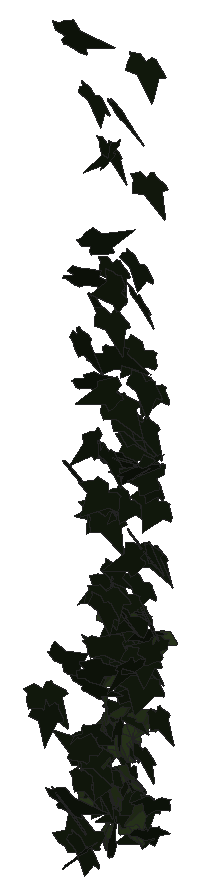
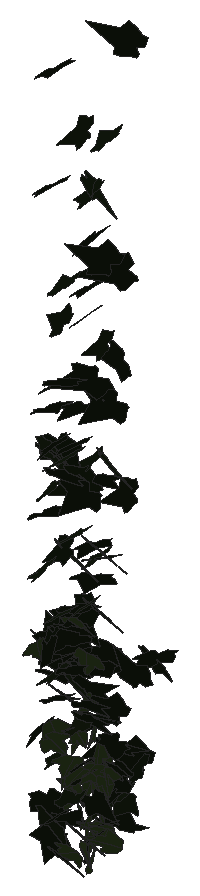
# SketchUp Ruby script. Lengths in inches.
U = 1.inch
M = Sketchup.active_model
def pt(a) = Geom::Point3d.new(a.map { |v| v * U })
def face(e, loops, mat)
  f = e.add_face(loops[0].map { |a| pt(a) })
  loops[1..].each { |l| e.add_face(l.map { |a| pt(a) }).erase! }
  f.material = f.back_material = mat if mat
  f
end
# faces: each face lists its corners as indices into pts; further lists are holes
def faces(e, pts, list, mat = nil) = list.each { |f| face(e, (f[0].is_a?(Array) ? f : [f]).map { |l| l.map { |i| pts[i] } }, mat) }
# xy, xz, yz: faces in a plane at the given z, y or x. An outline is a flat list of corners, or four numbers for a rectangle; further outlines are holes
def ring(l) = l.size == 4 ? [[l[0], l[1]], [l[2], l[1]], [l[2], l[3]], [l[0], l[3]]] : l.each_slice(2).to_a
def flat(e, list, mat, &to3) = list.each { |f| face(e, (f[0].is_a?(Array) ? f : [f]).map { |l| ring(l).map { |u, v| to3.(u, v) } }, mat) }
def xy(e, z, list, mat = nil) = flat(e, list, mat) { |x, y| [x, y, z] }
def xz(e, y, list, mat = nil) = flat(e, list, mat) { |x, z| [x, y, z] }
def yz(e, x, list, mat = nil) = flat(e, list, mat) { |y, z| [x, y, z] }
def lines(e, pts, list) = list.each { |a, b| e.add_line(pt(pts[a]), pt(pts[b])) }
# prism: a flat outline (further loops are holes) pulled along v
def prism(e, loops, v, mat = nil)
  f = face(e, loops, mat); d = Geom::Vector3d.new(v.map { |x| x * U })
  f.pushpull(f.normal.samedirection?(d) ? d.length : -d.length)
end
def box(e, o, s, mat = nil) = prism(e, [[o, [o[0] + s[0], o[1], o[2]], [o[0] + s[0], o[1] + s[1], o[2]], [o[0], o[1] + s[1], o[2]]]], [0, 0, s[2]], mat)
def at(x, y, z, deg = 0) = Geom::Transformation.translation(pt([x, y, z])) * Geom::Transformation.rotation(ORIGIN, Z_AXIS, deg.degrees)
def axes(o, x, y, z) = Geom::Transformation.new([*x, 0, *y, 0, *z, 0, *pt(o).to_a, 1])
def part(name) = M.definitions.add(name)
# library, detail: a bought-in or finely detailed component or shape, given as its bounding box
def library(name, o, s) = part(name).tap { |d| box(d.entities, o, s) }
def detail(e, o, s) = box(e.add_group.entities, o, s)
def put(e, d, t, mat = nil) = e.add_instance(d, t).tap { |i| i.material = mat if mat }
def group(e, t, mat = nil) = e.add_group.tap { |g| g.transformation = t; g.material = mat if mat }.entities
root = M.entities
M.materials.add("1026 AP 7946 SUNNY SIDE UP").color = [254, 231, 186]
M.materials.add("efeu1").color = [18, 25, 13]
M.materials.add("efeu2").color = [43, 57, 29]
c1 = part("ivyleaf_9")
p = [[1.54,2.16,1.25],[1.36,2.04,1.19],[-0.21,0.99,0.68],[-0.71,1.11,0.82],[-0.85,0.86,0.67],[-0.8,0.17,0.21],
  [-0.9,-0.01,0.1],[-0.67,-0.16,-0.02],[-0.08,-0.08,-0.05],[-0.03,-0.6,-0.4],[0.65,-0.88,-0.66],[0.83,-0.6,-0.49],
  [1.29,-0.42,-0.43],[1.8125,-0.07,-0.26],[1.21,0.44,0.15]]
faces(c1.entities,p,[[0,1,2,3,4,5,6,7,8,9,10,11,12,13,14]],"efeu1")
c2 = part("ivyleaf_10")
p = [[0,0.5,-0.03],[-0.0625,2.02,-0.43],[-0.19,2.01,-0.46],[-0.54,1.05,-0.29],[-0.52,0.625,-0.18],[-0.83,0.76,-0.28],
  [-1.16,0.64,-0.33],[-1.15,0.33,-0.24],[-0.77,-0.39,0.02],[-0.3,-0.51,0.16],[0.04,-0.48,0.23],[-0.02,2.01,-0.4375],
  [-0.06,2.01,-0.43],[0.04,-0.49,0.23],[0.67,-0.49,0.14],[1.38,0.36,-0.2],[1.375,0.51,-0.24],[0.81,0.65,-0.19],
  [0.62,0.59,-0.15],[0.6,1.09,-0.28],[0.5,1.23,-0.31]]
faces(c2.entities,p,[[0,1,2,3,4,5,6,7,8,9,10],[11,12,0,13,14,15,16,17,18,19,20]],"efeu2")
put(root,c1,axes([142.15,210.58,305.85],[0.56182,-0.24901,0.07476],[0.06155,-0.07277,-0.44748],[0.40379,0.35755,-0.03581]),"1026 AP 7946 SUNNY SIDE UP")
put(root,c1,axes([142.23,210.13,298.04],[-0.16216,0.04848,0.41407],[0.43975,-0.29098,0.10846],[0.45969,0.29546,0.04232]),"1026 AP 7946 SUNNY SIDE UP")
put(root,c2,axes([142.22,211.47,291.9],[-0.09766,-0.0032,0.39572],[0.44557,0.26235,0.05098],[-0.40784,0.28739,-0.03905]),"1026 AP 7946 SUNNY SIDE UP")
put(root,c1,axes([142.65,211.97,303.67],[-0.39464,-0.2842,0.1348],[0.01517,-0.17659,-0.37252],[0.4928,-0.22216,0.11942]),"1026 AP 7946 SUNNY SIDE UP")
put(root,c1,axes([142.35,211.77,320.69],[0.01203,-0.38419,0.25002],[0.09974,-0.24162,-0.394],[0.7094,0.04049,0.05115]),"1026 AP 7946 SUNNY SIDE UP")
put(root,c2,axes([142.7,211.37,294.5625],[-0.1224,-0.38129,-0.03837],[0.00721,0.03487,-0.4007],[0.60204,-0.07794,-0.00301]),"1026 AP 7946 SUNNY SIDE UP")
put(root,c1,axes([142.92,211.75,293.68],[-0.17105,0.24532,-0.2627],[0.04053,-0.26199,-0.27106],[-0.5565,-0.09449,0.061]),"1026 AP 7946 SUNNY SIDE UP")
put(root,c1,axes([142.77,211.86,292.65],[-0.37015,-0.23425,0.17707],[-0.05585,-0.19795,-0.32668],[0.45467,-0.21501,0.10402]),"1026 AP 7946 SUNNY SIDE UP")
put(root,c1,axes([143,212.11,297.29],[-0.56008,-0.05361,0.10937],[-0.12492,-0.14335,-0.34901],[0.13974,-0.34301,0.12636]),"1026 AP 7946 SUNNY SIDE UP")
put(root,c1,axes([143.2,211.61,303.96],[-0.52628,0.24654,0.09131],[-0.15815,0.00943,-0.42496],[-0.37958,-0.34575,0.05046]),"1026 AP 7946 SUNNY SIDE UP")
put(root,c1,axes([142.41,211.6875,312.36],[0.43938,-0.32096,0.01476],[-0.01385,-0.02904,-0.43778],[0.50513,0.27839,-0.02484]),"1026 AP 7946 SUNNY SIDE UP")
put(root,c1,axes([142.96,212.32,297.8],[-0.52887,-0.16853,0.03592],[-0.02311,-0.05023,-0.38586],[0.26994,-0.3345,0.03735]),"1026 AP 7946 SUNNY SIDE UP")
put(root,c2,axes([143.05,211.21,294.29],[-0.49013,0.10462,0.18163],[-0.27752,0.02416,-0.33723],[-0.16241,-0.357,0.02813]),"1026 AP 7946 SUNNY SIDE UP")
put(root,c2,axes([142.87,211.92,294.82],[0.22328,0.24384,-0.27449],[-0.17662,-0.24385,-0.29149],[-0.54146,0.18009,-0.01811]),"1026 AP 7946 SUNNY SIDE UP")
put(root,c1,axes([143.05,212.14,297.15],[-0.57967,-0.07156,-0.00169],[0.01229,-0.03379,-0.38542],[0.11186,-0.3671,0.03356]),"1026 AP 7946 SUNNY SIDE UP")
put(root,c1,axes([142.94,211.03,294.74],[-0.5539,-0.10903,-0.12035],[0.18925,0.00271,-0.37848],[0.1642,-0.37092,0.03025]),"1026 AP 7946 SUNNY SIDE UP")
put(root,c1,axes([143.15,210.9,307.13],[-0.58674,0.18478,-0.14982],[0.17748,-0.10077,-0.42777],[-0.32553,-0.38799,0.03682]),"1026 AP 7946 SUNNY SIDE UP")
put(root,c2,axes([142.49,211.59,292.5],[0.05579,-0.14515,-0.35271],[0.58133,0.04364,0.02072],[0.05071,-0.3406,0.15058]),"1026 AP 7946 SUNNY SIDE UP")
put(root,c1,axes([143.24,211.65,318.73],[-0.47623,0.33135,-0.12901],[0.10289,-0.11211,-0.46233],[-0.54848,-0.30874,0.02529]),"1026 AP 7946 SUNNY SIDE UP")
put(root,c1,axes([142.47,210.72,311.3],[-0.00696,-0.0332,-0.47585],[0.72787,0.00217,-0.00472],[0.00393,-0.46173,0.03147]),"1026 AP 7946 SUNNY SIDE UP")
put(root,c2,axes([143.09,211.16,292.66],[0.23101,-0.30684,-0.17315],[-0.10165,0.15342,-0.3495],[0.53931,0.16035,0.00829]),"1026 AP 7946 SUNNY SIDE UP")
put(root,c2,axes([143.02,211.08,294.53],[0.09477,0.20416,-0.33964],[-0.15232,-0.31635,-0.22114],[-0.59201,0.11408,0.00253]),"1026 AP 7946 SUNNY SIDE UP")
put(root,c1,axes([142.97,211.62,292.02],[-0.17279,-0.25937,0.22693],[-0.09181,-0.21523,-0.29042],[0.52865,-0.12216,0.02373]),"1026 AP 7946 SUNNY SIDE UP")
put(root,c1,axes([142.71,210.875,309.56],[0.55799,0.25387,0.14941],[0.21938,0.05084,-0.44751],[-0.40273,0.37943,-0.03676]),"1026 AP 7946 SUNNY SIDE UP")
put(root,c1,axes([142.39,210.16,323.9],[0.25932,-0.02808,0.45404],[0.61742,-0.20636,-0.16606],[0.31836,0.42309,-0.04779]),"1026 AP 7946 SUNNY SIDE UP")
put(root,c1,axes([143.47,209.95,294.84],[-0.1309,0.16315,0.34222],[-0.53841,0.09301,-0.1353],[-0.21736,-0.32866,0.12904]),"1026 AP 7946 SUNNY SIDE UP")
put(root,c2,axes([143.02,211.31,295.42],[0.00064,-0.32487,-0.19179],[0.05825,0.18345,-0.33193],[0.58442,-0.01793,0.0333]),"1026 AP 7946 SUNNY SIDE UP")
put(root,c1,axes([142.81,210.5625,293.5],[0.18628,-0.37561,-0.22452],[-0.13524,0.19889,-0.40408],[0.6676,0.1451,-0.01921]),"1026 AP 7946 SUNNY SIDE UP")
put(root,c1,axes([142.68,212.14,318.62],[0.28861,-0.40925,0.05953],[0.01196,-0.06241,-0.46204],[0.65029,0.18278,-0.01792]),"1026 AP 7946 SUNNY SIDE UP")
put(root,c1,axes([143.48,211.49,297.87],[-0.00745,0.14018,0.37491],[-0.57798,0.11785,-0.05112],[-0.20134,-0.3435,0.13288]),"1026 AP 7946 SUNNY SIDE UP")
put(root,c1,axes([142.54,210.51,294.08],[0.35755,0.10931,-0.31997],[0.41372,0.16786,0.25977],[0.31279,-0.34697,0.02216]),"1026 AP 7946 SUNNY SIDE UP")
put(root,c1,axes([142.8,212.28,313.67],[0.11444,-0.43428,-0.01193],[-0.00085,0.00915,-0.45357],[0.68301,0.07278,0.00143]),"1026 AP 7946 SUNNY SIDE UP")
put(root,c1,axes([142.55,210.9375,296.875],[0.19017,-0.11545,0.38404],[0.52678,-0.17077,-0.16716],[0.31664,0.35344,0.04745]),"1026 AP 7946 SUNNY SIDE UP")
put(root,c2,axes([143.12,210.79,294.86],[0.20138,-0.37363,0.07668],[0.01933,-0.07667,-0.40712],[0.59939,0.128,-0.01264]),"1026 AP 7946 SUNNY SIDE UP")
put(root,c1,axes([143.41,211.23,301.14],[-0.6215,0.11195,-0.05232],[0.05893,-0.05534,-0.42124],[-0.18452,-0.39472,0.04168]),"1026 AP 7946 SUNNY SIDE UP")
put(root,c1,axes([142.88,208.1875,298.01],[0.02358,-0.36781,-0.3025],[0.06117,0.29167,-0.3753],[0.73546,-0.01246,0.04091]),"1026 AP 7946 SUNNY SIDE UP")
put(root,c2,axes([143.05,211.95,299.5],[0.61704,0.00807,0.06382],[0.09665,0.01891,-0.40384],[-0.01715,0.39682,0.02028]),"1026 AP 7946 SUNNY SIDE UP")
put(root,c2,axes([143.29,211.15,293.8],[0.07042,-0.38256,0.03993],[0.0033,-0.04096,-0.39703],[0.60496,0.04475,-0.00248]),"1026 AP 7946 SUNNY SIDE UP")
put(root,c1,axes([143.04,210.33,295.3],[0.09394,0.01372,-0.42097],[-0.04812,0.41204,0.01206],[0.64121,0.02891,0.06258]),"1026 AP 7946 SUNNY SIDE UP")
put(root,c2,axes([143.34,211.47,292.61],[-0.1965,0.34061,0.13927],[-0.15386,0.10455,-0.36923],[-0.55413,-0.14981,0.05313]),"1026 AP 7946 SUNNY SIDE UP")
put(root,c2,axes([143.42,211.39,290.625],[-0.24085,0.33001,-0.08377],[-0.04459,0.07854,0.3752],[0.53329,0.15561,-0.00646]),"1026 AP 7946 SUNNY SIDE UP")
put(root,c2,axes([143.34,211.79,297.35],[0.05907,0.14871,-0.37206],[-0.13408,-0.35182,-0.16006],[-0.60058,0.09317,-0.00086]),"1026 AP 7946 SUNNY SIDE UP")
put(root,c2,axes([143.36,211.16,296.12],[0.15168,-0.19433,-0.35009],[0.01038,0.34967,-0.20269],[0.61395,0.0421,0.08992]),"1026 AP 7946 SUNNY SIDE UP")
put(root,c1,axes([142.94,210.93,315.14],[0.05738,-0.02267,0.47504],[0.68454,0.15606,-0.02667],[-0.24227,0.43558,0.03716]),"1026 AP 7946 SUNNY SIDE UP")
put(root,c1,axes([143.63,209.57,291.35],[-0.68018,-0.12224,0.10938],[0.14472,0.06593,0.46186],[-0.21032,0.44067,-0.03592]),"1026 AP 7946 SUNNY SIDE UP")
put(root,c1,axes([143.17,212.13,294.59],[-0.0023,-0.40131,0.02534],[0.00114,-0.02688,-0.41359],[0.63243,-0.00141,0.00084]),"1026 AP 7946 SUNNY SIDE UP")
put(root,c2,axes([143.36,211.82,291.44],[0.24741,-0.30684,0.09887],[0.04404,-0.09531,-0.35532],[0.50443,0.15882,-0.01748]),"1026 AP 7946 SUNNY SIDE UP")
put(root,c1,axes([143.18,211.78,306.14],[0.65164,0.12028,0.00081],[0.01776,-0.03854,-0.44285],[-0.1883,0.41262,-0.03896]),"1026 AP 7946 SUNNY SIDE UP")
put(root,c1,axes([143.17,211.19,292.78],[0.1197,-0.35243,0.14097],[0.06544,-0.13298,-0.37202],[0.592,0.08596,0.01262]),"1026 AP 7946 SUNNY SIDE UP")
put(root,c1,axes([143.21,211.35,303.8125],[-0.00117,-0.37081,-0.18904],[0.06235,0.18049,-0.37922],[0.64609,-0.01809,0.03625]),"1026 AP 7946 SUNNY SIDE UP")
put(root,c1,axes([143.17,211.19,298.89],[-0.03985,-0.18991,-0.3936],[0.14811,0.3697,-0.19414],[0.65277,-0.09548,0.02002]),"1026 AP 7946 SUNNY SIDE UP")
put(root,c1,axes([143.27,211.92,301.38],[-0.02768,-0.38086,0.15386],[0.02233,-0.15213,-0.39315],[0.64414,-0.01109,0.02024]),"1026 AP 7946 SUNNY SIDE UP")
put(root,c1,axes([143.35,207.87,297.5625],[-0.48477,-0.05324,-0.34856],[0.53801,-0.04,-0.31522],[0.00941,-0.45577,0.06566]),"1026 AP 7946 SUNNY SIDE UP")
put(root,c1,axes([143.3,212.15,296.54],[-0.16051,-0.26235,0.30002],[0.12956,-0.30999,-0.25843],[0.60435,-0.00322,0.13509]),"1026 AP 7946 SUNNY SIDE UP")
put(root,c1,axes([143,209.87,314.39],[0.59073,0.10384,0.29118],[0.43649,0.05325,-0.40078],[-0.18122,0.46676,-0.01615]),"1026 AP 7946 SUNNY SIDE UP")
put(root,c1,axes([143.34,211.8,294.99],[0.18955,-0.34113,-0.14456],[-0.03364,0.13888,-0.37106],[0.57787,0.11998,0.02582]),"1026 AP 7946 SUNNY SIDE UP")
put(root,c1,axes([143.22,211.3125,310.58],[0.03452,0.02512,-0.47349],[0.27578,0.42512,0.03505],[0.66941,-0.17643,0.00998]),"1026 AP 7946 SUNNY SIDE UP")
put(root,c2,axes([143.36,211.2,294.46],[0.00923,-0.15631,-0.37194],[0.39566,0.27798,-0.11844],[0.47387,-0.22906,0.10613]),"1026 AP 7946 SUNNY SIDE UP")
put(root,c1,axes([144.04,210.76,309.57],[-0.64741,0.16256,0.03989],[-0.07717,-0.02175,-0.45446],[-0.25083,-0.41289,0.03685]),"1026 AP 7946 SUNNY SIDE UP")
put(root,c1,axes([143.23,208.72,293.48],[0.41095,-0.33522,0.15033],[0.0966,-0.13891,-0.43723],[0.56792,0.2662,-0.0344]),"1026 AP 7946 SUNNY SIDE UP")
put(root,c1,axes([143.58,212.24,304.3],[-0.21193,-0.31969,0.23678],[0.00341,-0.24538,-0.34899],[0.62077,-0.1078,0.08275]),"1026 AP 7946 SUNNY SIDE UP")
put(root,c1,axes([143.47,210.41,294.65],[0.0249,-0.33405,-0.21233],[0.01873,0.20469,-0.3428],[0.61535,0.00728,0.01903]),"1026 AP 7946 SUNNY SIDE UP")
put(root,c1,axes([143.53,212.11,299.79],[-0.06043,-0.36397,-0.15254],[0.03457,0.14447,-0.37614],[0.61566,-0.04384,0.00615]),"1026 AP 7946 SUNNY SIDE UP")
put(root,c1,axes([144.04,211.71,298.23],[-0.46982,0.26744,-0.02948],[0.00484,-0.04163,-0.41228],[-0.42316,-0.29741,0.02801]),"1026 AP 7946 SUNNY SIDE UP")
put(root,c1,axes([143.82,212.07,298.78],[-0.41964,-0.27726,0.09473],[-0.08011,-0.08062,-0.39646],[0.45306,-0.27106,0.01764]),"1026 AP 7946 SUNNY SIDE UP")
put(root,c2,axes([143.94,210.41,291.36],[-0.07201,0.18956,0.33032],[-0.32142,0.25601,-0.18513],[-0.48786,-0.19665,0.07321]),"1026 AP 7946 SUNNY SIDE UP")
put(root,c1,axes([143.375,211.64,320.72],[0.52941,-0.32928,-0.01128],[-0.02975,-0.00637,-0.48485],[0.5171,0.33675,-0.01635]),"1026 AP 7946 SUNNY SIDE UP")
put(root,c1,axes([144.13,211.48,291.93],[-0.52827,0.18761,0.04887],[-0.08806,-0.0055,-0.39509],[-0.29083,-0.33911,0.03086]),"1026 AP 7946 SUNNY SIDE UP")
put(root,c2,axes([143.59,211.68,294.49],[0.31962,0.25173,0.20501],[0.11725,0.19036,-0.32778],[-0.48932,0.21004,0.05537]),"1026 AP 7946 SUNNY SIDE UP")
put(root,c1,axes([143.41,211.38,306.26],[0.64576,0.06142,0.13458],[0.17585,0.1121,-0.41696],[-0.14273,0.41601,0.09515]),"1026 AP 7946 SUNNY SIDE UP")
put(root,c2,axes([143.79,210.79,294.1875],[0.13115,-0.30077,0.21082],[0.12537,-0.19152,-0.32191],[0.55967,0.11339,0.02271]),"1026 AP 7946 SUNNY SIDE UP")
put(root,c2,axes([143.875,210.47,291.43],[-0.11108,0.33213,0.16192],[-0.11244,0.14262,-0.34693],[-0.56543,-0.09361,0.03718]),"1026 AP 7946 SUNNY SIDE UP")
put(root,c2,axes([143.92,211.51,296.02],[-0.04327,-0.35273,0.17459],[0.03837,-0.17311,-0.36381],[0.6155,-0.014,0.03495]),"1026 AP 7946 SUNNY SIDE UP")
put(root,c2,axes([143.77,211.93,295.02],[0.30164,0.32188,0.10855],[0.04961,0.10148,-0.38464],[-0.52934,0.19293,0.02581]),"1026 AP 7946 SUNNY SIDE UP")
put(root,c1,axes([143.63,211.87,307.98],[0.13886,-0.37343,-0.16441],[0.04527,0.16654,-0.38926],[0.63565,0.06972,0.06364]),"1026 AP 7946 SUNNY SIDE UP")
put(root,c1,axes([143.96,210.73,290.67],[-0.00409,-0.16012,0.38091],[0.20303,0.35087,0.15914],[-0.60155,0.11951,0.05112]),"1026 AP 7946 SUNNY SIDE UP")
put(root,c1,axes([143.62,211,306.79],[0.16267,-0.39106,0.14458],[0.04113,-0.1405,-0.41742],[0.6532,0.10623,-0.00972]),"1026 AP 7946 SUNNY SIDE UP")
put(root,c1,axes([143.93,210.55,293.99],[-0.33185,-0.32163,0.04004],[-0.01006,-0.04441,-0.39609],[0.50966,-0.2103,0.01826]),"1026 AP 7946 SUNNY SIDE UP")
put(root,c1,axes([144.17,212.27,306.79],[-0.62799,-0.11032,0.02007],[-0.01241,-0.04657,-0.42485],[0.17588,-0.39717,0.04171]),"1026 AP 7946 SUNNY SIDE UP")
put(root,c2,axes([143.76,211.42,292.41],[-0.04906,0.01337,-0.36949],[0.15961,-0.34507,-0.02436],[-0.54144,-0.10293,0.0263]),"1026 AP 7946 SUNNY SIDE UP")
put(root,c1,axes([144.1,210.28,305.67],[-0.477,-0.26059,0.10281],[-0.0996,-0.0815,-0.41196],[0.42819,-0.30926,0.01871]),"1026 AP 7946 SUNNY SIDE UP")
put(root,c1,axes([143.76,211.64,299.98],[0.54368,0.2194,0.03463],[0.06102,-0.00081,-0.42129],[-0.34334,0.34728,-0.02002]),"1026 AP 7946 SUNNY SIDE UP")
put(root,c1,axes([143.63,211.55,296.22],[0.18287,-0.30156,-0.24316],[0.10539,0.25726,-0.30531],[0.59118,0.04742,0.12964]),"1026 AP 7946 SUNNY SIDE UP")
put(root,c1,axes([143.53,209.875,298.38],[0.25504,0.19127,-0.36868],[0.22544,0.33475,0.25246],[0.5985,-0.2076,0.06201]),"1026 AP 7946 SUNNY SIDE UP")
put(root,c1,axes([144.07,212.36,310.57],[-0.45422,-0.30101,0.09668],[-0.0282,-0.11366,-0.42536],[0.49579,-0.28224,0.06438]),"1026 AP 7946 SUNNY SIDE UP")
put(root,c2,axes([144.05,211.98,294.6],[-0.31746,0.32632,0.05372],[-0.09415,0.02179,-0.39312],[-0.51055,-0.20692,0.03909]),"1026 AP 7946 SUNNY SIDE UP")
put(root,c1,axes([144.29,211.59,292.21],[-0.56855,-0.12977,0.07206],[0.0977,0.03602,0.39576],[-0.21083,0.36666,-0.01094]),"1026 AP 7946 SUNNY SIDE UP")
put(root,c1,axes([143.74,211.91,307.49],[0.35585,-0.29997,-0.19565],[-0.02513,0.21448,-0.37071],[0.55626,0.20159,0.10841]),"1026 AP 7946 SUNNY SIDE UP")
put(root,c1,axes([144.26,211.99,297.64],[-0.60814,0.00536,-0.1049],[0.15391,-0.09289,-0.38844],[-0.04513,-0.38901,0.08891]),"1026 AP 7946 SUNNY SIDE UP")
put(root,c2,axes([143.8125,211.89,291.22],[-0.40933,-0.02938,-0.2753],[0.37481,-0.19685,-0.2182],[-0.19495,-0.31677,0.15855]),"1026 AP 7946 SUNNY SIDE UP")
put(root,c1,axes([143.75,210.89,300.75],[0.62833,-0.1692,-0.02395],[-0.05597,-0.02713,-0.44541],[0.26244,0.3993,-0.03764]),"1026 AP 7946 SUNNY SIDE UP")
put(root,c1,axes([143.5,208.44,293.53],[0.27721,-0.09804,0.43974],[0.61155,-0.1778,-0.20833],[0.31847,0.42678,0.01729]),"1026 AP 7946 SUNNY SIDE UP")
put(root,c1,axes([144.125,211.39,300.91],[-0.35984,-0.33719,0.01263],[0.01939,-0.02547,-0.41921],[0.53032,-0.22786,0.0239]),"1026 AP 7946 SUNNY SIDE UP")
put(root,c2,axes([144.14,210.46,293.49],[-0.48053,0.21938,-0.02901],[0.01038,-0.04108,-0.3866],[-0.34788,-0.30425,0.02854]),"1026 AP 7946 SUNNY SIDE UP")
put(root,c1,axes([144.1,211.6,293.67],[-0.39218,0.02697,-0.28347],[0.41071,-0.09911,-0.25436],[-0.14324,-0.35803,0.04679]),"1026 AP 7946 SUNNY SIDE UP")
put(root,c1,axes([144.1,211.78,300.23],[-0.443,-0.27639,-0.11732],[0.19044,0.03521,-0.40206],[0.42872,-0.30125,0.05738]),"1026 AP 7946 SUNNY SIDE UP")
put(root,c1,axes([144.04,212.39,300.98],[-0.14401,-0.34802,0.18194],[0.03034,-0.18721,-0.36675],[0.61432,-0.07234,0.06076]),"1026 AP 7946 SUNNY SIDE UP")
put(root,c2,axes([143.9,211.375,300.125],[-0.43751,0.06497,-0.28576],[0.40631,-0.10693,-0.29306],[-0.18998,-0.37833,0.0313]),"1026 AP 7946 SUNNY SIDE UP")
put(root,c1,axes([144.02,211.82,293.19],[-0.17282,-0.23563,0.28088],[0.16865,-0.29474,-0.21853],[0.54261,0.01657,0.15738]),"1026 AP 7946 SUNNY SIDE UP")
put(root,c1,axes([144.38,212.34,297.49],[-0.40866,-0.19355,0.20423],[-0.16216,-0.18626,-0.32592],[0.40568,-0.26943,0.07545]),"1026 AP 7946 SUNNY SIDE UP")
put(root,c1,axes([144.55,211.98,291.03],[-0.51861,0.12623,0.03316],[-0.06088,-0.01335,-0.36289],[-0.19529,-0.33105,0.02505]),"1026 AP 7946 SUNNY SIDE UP")
put(root,c1,axes([144.54,211.03,300.34],[0.19763,0.12837,-0.40784],[-0.33181,-0.33766,-0.18345],[-0.56531,0.24307,-0.0349]),"1026 AP 7946 SUNNY SIDE UP")
put(root,c1,axes([144,211.01,309.02],[0.02749,-0.34486,-0.27463],[0.14416,0.26181,-0.34372],[0.66814,-0.0423,0.08546]),"1026 AP 7946 SUNNY SIDE UP")
put(root,c1,axes([144.11,212.09,314.26],[-0.08494,-0.35662,0.26364],[0.06681,-0.26288,-0.3668],[0.68882,-0.01848,0.06808]),"1026 AP 7946 SUNNY SIDE UP")
put(root,c1,axes([144.1,210.93,295.8],[-0.12626,-0.09148,-0.36741],[0.5461,-0.13853,-0.04483],[-0.18978,-0.33776,0.11544]),"1026 AP 7946 SUNNY SIDE UP")
put(root,c1,axes([144.44,208.06,291.7],[0.12501,0.40456,0.24098],[0.09231,0.2244,-0.42324],[-0.72718,0.09803,-0.0123]),"1026 AP 7946 SUNNY SIDE UP")
put(root,c1,axes([144,212.18,312.85],[0.21724,-0.34009,0.24987],[0.11338,-0.23428,-0.37909],[0.64875,0.15482,-0.01742]),"1026 AP 7946 SUNNY SIDE UP")
put(root,c1,axes([144.21,210.18,301.6],[-0.23716,-0.33715,-0.20514],[0.15855,0.17064,-0.37896],[0.59335,-0.18035,0.01927]),"1026 AP 7946 SUNNY SIDE UP")
put(root,c2,axes([143.95,211.42,293.43],[-0.01049,0.00185,0.40702],[0.60873,-0.07885,0.00665],[0.12402,0.38719,0.00177]),"1026 AP 7946 SUNNY SIDE UP")
put(root,c2,axes([144.34,210.73,295.29],[-0.03131,0.36957,0.08826],[-0.00311,0.08359,-0.38079],[-0.59579,-0.01986,-0.00265]),"1026 AP 7946 SUNNY SIDE UP")
put(root,c2,axes([144.61,212.13,295.65],[-0.29737,-0.22425,0.24212],[-0.08989,-0.24615,-0.28923],[0.5043,-0.17611,0.09122]),"1026 AP 7946 SUNNY SIDE UP")
put(root,c1,axes([144.29,208.76,291.77],[-0.05776,-0.37429,0.30701],[0.06397,-0.30236,-0.38509],[0.75167,-0.00303,0.05636]),"1026 AP 7946 SUNNY SIDE UP")
put(root,c2,axes([144.66,211.91,296.05],[-0.25669,-0.3343,0.10749],[-0.03439,-0.10725,-0.38293],[0.55049,-0.16258,0.0262]),"1026 AP 7946 SUNNY SIDE UP")
put(root,c1,axes([144.96,211.03,302.93],[-0.61897,0.24894,0.00023],[-0.03049,-0.03288,-0.4784],[-0.39025,-0.39227,0.03701]),"1026 AP 7946 SUNNY SIDE UP")
put(root,c1,axes([144.23,211.59,303.35],[0.50508,-0.24826,-0.01647],[-0.04627,-0.0143,-0.41723],[0.38829,0.32123,-0.0283]),"1026 AP 7946 SUNNY SIDE UP")
put(root,c1,axes([144.33,211.91,298.43],[0.32878,-0.33092,-0.09574],[-0.02787,0.09606,-0.40105],[0.53896,0.20684,0.03766]),"1026 AP 7946 SUNNY SIDE UP")
put(root,c1,axes([144.6,212.33,309.3],[-0.28727,-0.37385,0.0898],[-0.00972,-0.096,-0.42764],[0.6043,-0.17926,0.03581]),"1026 AP 7946 SUNNY SIDE UP")
put(root,c1,axes([144.43,212,307.8],[0.16702,-0.36754,-0.1615],[-0.05123,0.15154,-0.39311],[0.62492,0.11066,0.01094]),"1026 AP 7946 SUNNY SIDE UP")
put(root,c1,axes([144.6,211.59,299.43],[0.40698,0.28802,0.04878],[0.07118,0.02071,-0.39828],[-0.45299,0.26202,-0.01875]),"1026 AP 7946 SUNNY SIDE UP")
put(root,c1,axes([144.54,211.99,292.41],[-0.03482,-0.37062,0.06127],[-0.00031,-0.06168,-0.38284],[0.59075,-0.02187,0.00341]),"1026 AP 7946 SUNNY SIDE UP")
put(root,c1,axes([144.86,210.83,298.63],[-0.15695,0.22483,-0.39716],[0.21194,-0.36278,-0.2552],[-0.67079,-0.16723,0.0123]),"1026 AP 7946 SUNNY SIDE UP")
put(root,c1,axes([144.57,209.94,313.23],[0.04188,-0.44967,-0.05689],[0.00974,0.05311,-0.46365],[0.71184,0.02573,0.00969]),"1026 AP 7946 SUNNY SIDE UP")
put(root,c1,axes([145.11,211.54,292.26],[-0.18518,0.39705,-0.06291],[0.0093,-0.06426,-0.42683],[-0.63214,-0.11726,0.01215]),"1026 AP 7946 SUNNY SIDE UP")
put(root,c1,axes([144.76,211.54,298.63],[-0.22743,-0.34558,-0.07979],[0.08687,0.05849,-0.38453],[0.54937,-0.15231,0.02777]),"1026 AP 7946 SUNNY SIDE UP")
put(root,c1,axes([144.86,211.56,291.43],[0.34859,0.27996,-0.04612],[-0.00931,-0.05425,-0.36701],[-0.44611,0.21989,-0.02838]),"1026 AP 7946 SUNNY SIDE UP")
put(root,c1,axes([144.7,211.78,322.89],[-0.04807,-0.46296,-0.01431],[0.01249,0.01076,-0.47786],[0.72807,-0.03075,0.00725]),"1026 AP 7946 SUNNY SIDE UP")
put(root,c2,axes([144.97,211.11,292.39],[0.06856,0.0942,-0.39291],[-0.16588,-0.3674,-0.10791],[-0.59589,0.11311,-0.01516]),"1026 AP 7946 SUNNY SIDE UP")
put(root,c1,axes([144.82,212.05,305.59],[-0.10703,-0.29493,0.29202],[-0.02724,-0.28671,-0.31145],[0.64446,-0.0611,0.03533]),"1026 AP 7946 SUNNY SIDE UP")
put(root,c1,axes([144.66,211.87,302.76],[0.26625,-0.36001,-0.14776],[0.00033,0.15443,-0.40392],[0.60817,0.15752,0.06491]),"1026 AP 7946 SUNNY SIDE UP")
put(root,c1,axes([144.72,211.58,294.63],[0.16045,-0.3583,0.09526],[0.02365,-0.09394,-0.38418],[0.58218,0.10257,-0.01065]),"1026 AP 7946 SUNNY SIDE UP")
put(root,c1,axes([144.76,209.3,301.72],[0.02123,-0.38397,0.14443],[0.04806,-0.14111,-0.39586],[0.64213,0.02326,0.02485]),"1026 AP 7946 SUNNY SIDE UP")
put(root,c1,axes([144.97,212.08,304.78],[-0.29665,-0.37629,0.1331],[-0.0447,-0.13224,-0.43314],[0.62509,-0.18803,0.03219]),"1026 AP 7946 SUNNY SIDE UP")
put(root,c1,axes([145.13,209.74,314.51],[-0.22743,-0.11317,0.44566],[-0.32073,-0.38865,-0.17702],[0.62679,-0.23993,0.07112]),"1026 AP 7946 SUNNY SIDE UP")
put(root,c1,axes([144.75,211.93,299.84],[0.0277,-0.18658,0.3696],[0.0879,-0.3556,-0.19486],[0.63124,0.05771,0.01091]),"1026 AP 7946 SUNNY SIDE UP")
put(root,c1,axes([144.84,211.58,309.87],[-0.04192,-0.43268,0.09131],[-0.00325,-0.09114,-0.44711],[0.69526,-0.02651,0.00342]),"1026 AP 7946 SUNNY SIDE UP")
put(root,c1,axes([144.77,212.2,302.62],[0.26464,-0.37817,-0.02803],[-0.03091,0.01867,-0.42618],[0.59513,0.16913,-0.00968]),"1026 AP 7946 SUNNY SIDE UP")
put(root,c1,axes([144.78,211.77,318.11],[0.10293,-0.43784,-0.10289],[0.03615,0.10157,-0.45389],[0.70435,0.05877,0.03833]),"1026 AP 7946 SUNNY SIDE UP")
put(root,c1,axes([145.27,211.49,292.83],[0.08799,0.28416,-0.28174],[-0.06812,-0.27176,-0.29986],[-0.61816,0.0704,-0.00706]),"1026 AP 7946 SUNNY SIDE UP")
put(root,c1,axes([145.5625,211.43,299.13],[-0.41501,0.27691,0.1697],[-0.23961,0.07806,-0.38999],[-0.44495,-0.30031,0.05174]),"1026 AP 7946 SUNNY SIDE UP")
put(root,c1,axes([145.39,210.7,306.9],[-0.03322,0.43254,-0.21589],[-0.1044,-0.21281,-0.44169],[-0.75021,0.01046,0.07103]),"1026 AP 7946 SUNNY SIDE UP")
put(root,c1,axes([145.04,211.26,297.81],[-0.50312,-0.28746,-0.11332],[0.25398,-0.02433,-0.425],[0.41089,-0.33695,0.12394]),"1026 AP 7946 SUNNY SIDE UP")
put(root,c1,axes([145.68,211,306.48],[-0.5348,0.21844,0.25474],[-0.3731,0.08227,-0.4127],[-0.35838,-0.41163,0.04951]),"1026 AP 7946 SUNNY SIDE UP")
put(root,c1,axes([144.98,212.07,296.07],[0.19539,-0.31561,-0.19695],[-0.13664,0.16908,-0.34803],[0.5624,0.15073,-0.01614]),"1026 AP 7946 SUNNY SIDE UP")
put(root,c1,axes([145.51,211.02,306.92],[-0.26861,0.42949,-0.02389],[-0.0359,-0.03658,-0.47505],[-0.67559,-0.16882,0.03474]),"1026 AP 7946 SUNNY SIDE UP")
put(root,c2,axes([145.21,212.13,299.3],[0.16223,0.34524,-0.13158],[-0.11694,-0.11242,-0.36992],[-0.56798,0.12176,0.03858]),"1026 AP 7946 SUNNY SIDE UP")
